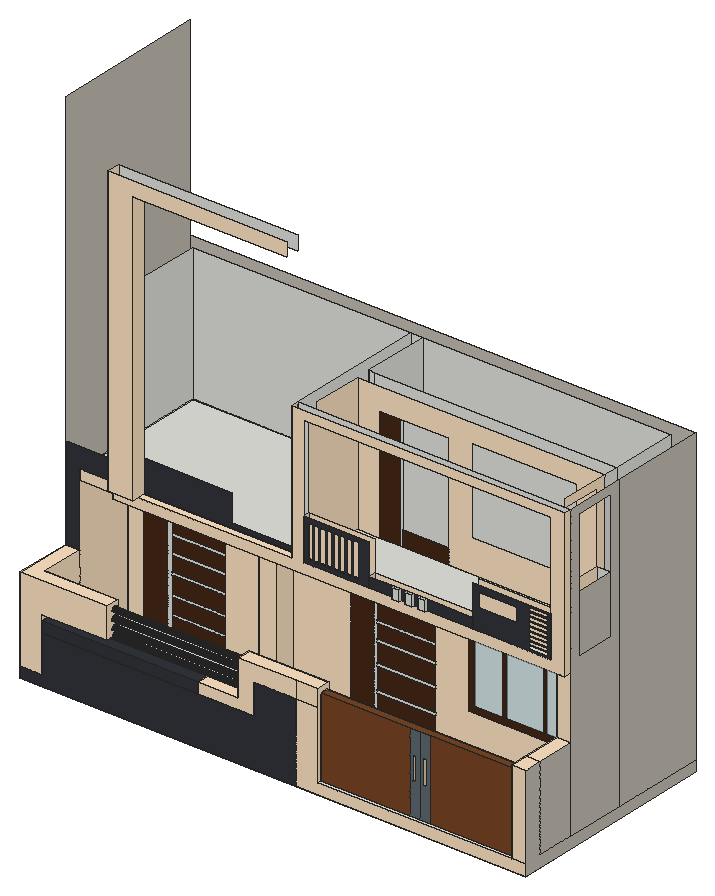
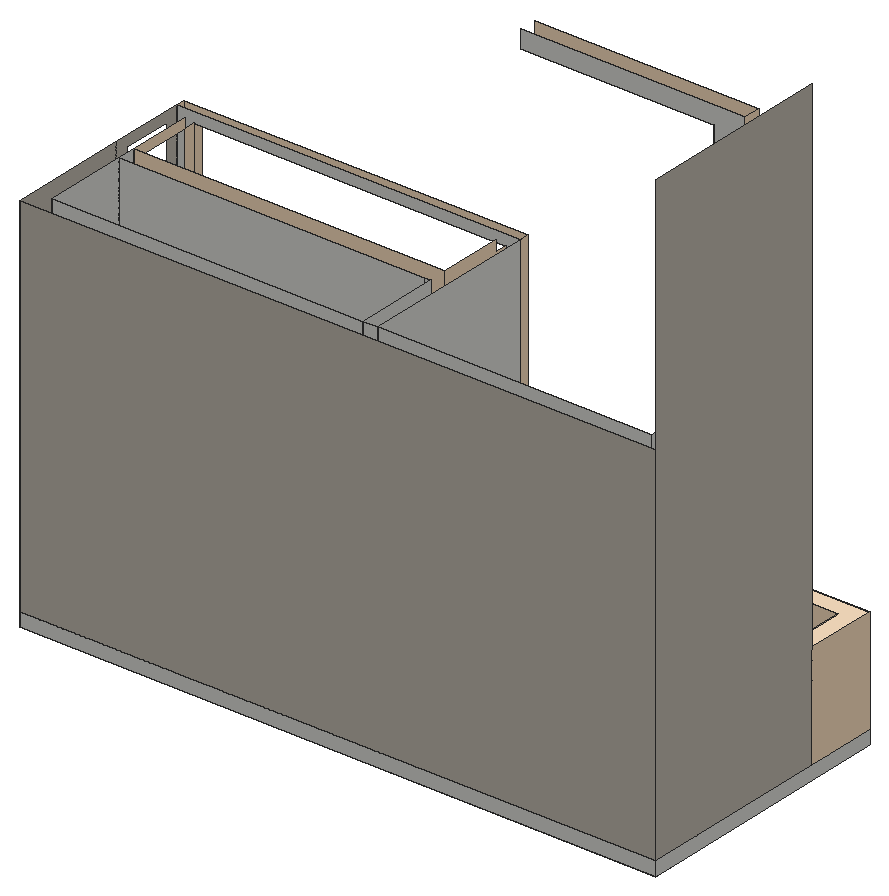
# SketchUp Ruby script. Lengths in inches.
U = 1.inch
M = Sketchup.active_model
def pt(a) = Geom::Point3d.new(a.map { |v| v * U })
def face(e, loops, mat)
  f = e.add_face(loops[0].map { |a| pt(a) })
  loops[1..].each { |l| e.add_face(l.map { |a| pt(a) }).erase! }
  f.material = f.back_material = mat if mat
  f
end
# faces: each face lists its corners as indices into pts; further lists are holes
def faces(e, pts, list, mat = nil) = list.each { |f| face(e, (f[0].is_a?(Array) ? f : [f]).map { |l| l.map { |i| pts[i] } }, mat) }
# xy, xz, yz: faces in a plane at the given z, y or x. An outline is a flat list of corners, or four numbers for a rectangle; further outlines are holes
def ring(l) = l.size == 4 ? [[l[0], l[1]], [l[2], l[1]], [l[2], l[3]], [l[0], l[3]]] : l.each_slice(2).to_a
def flat(e, list, mat, &to3) = list.each { |f| face(e, (f[0].is_a?(Array) ? f : [f]).map { |l| ring(l).map { |u, v| to3.(u, v) } }, mat) }
def xy(e, z, list, mat = nil) = flat(e, list, mat) { |x, y| [x, y, z] }
def xz(e, y, list, mat = nil) = flat(e, list, mat) { |x, z| [x, y, z] }
def yz(e, x, list, mat = nil) = flat(e, list, mat) { |y, z| [x, y, z] }
def lines(e, pts, list) = list.each { |a, b| e.add_line(pt(pts[a]), pt(pts[b])) }
# prism: a flat outline (further loops are holes) pulled along v
def prism(e, loops, v, mat = nil)
  f = face(e, loops, mat); d = Geom::Vector3d.new(v.map { |x| x * U })
  f.pushpull(f.normal.samedirection?(d) ? d.length : -d.length)
end
def box(e, o, s, mat = nil) = prism(e, [[o, [o[0] + s[0], o[1], o[2]], [o[0] + s[0], o[1] + s[1], o[2]], [o[0], o[1] + s[1], o[2]]]], [0, 0, s[2]], mat)
def at(x, y, z, deg = 0) = Geom::Transformation.translation(pt([x, y, z])) * Geom::Transformation.rotation(ORIGIN, Z_AXIS, deg.degrees)
def axes(o, x, y, z) = Geom::Transformation.new([*x, 0, *y, 0, *z, 0, *pt(o).to_a, 1])
def part(name) = M.definitions.add(name)
# library, detail: a bought-in or finely detailed component or shape, given as its bounding box
def library(name, o, s) = part(name).tap { |d| box(d.entities, o, s) }
def detail(e, o, s) = box(e.add_group.entities, o, s)
def put(e, d, t, mat = nil) = e.add_instance(d, t).tap { |i| i.material = mat if mat }
def group(e, t, mat = nil) = e.add_group.tap { |g| g.transformation = t; g.material = mat if mat }.entities
root = M.entities
M.materials.add("[0012_Bisque]").color = [255, 228, 196]
M.materials.add("[Color M08]").color = [30, 30, 30]
M.materials.add("[Field Rectangle Tile]").color = [196, 189, 179]
M.materials.add("[Formica Laminate Dark]").color = [50, 53, 60]
M.materials.add("[Formica Laminate Light]").color = [213, 189, 164]
M.materials.add("[Formica Speckled Grey]").color = [94, 105, 111]
M.materials.add("[Translucent Glass Safety]").color = [204, 235, 244]
M.materials["[Translucent Glass Safety]"].alpha = 0.5
M.materials.add("[Wood Veneer 01]").color = [68, 40, 21]
M.materials.add("[Wood Veneer 01]1").color = [120, 70, 37]
xy(root,0,[[24.6875,0,439.21,174.44]])
xy(root,9,[[24.6875,0,24.6875,46.73,36.15,46.73,36.15,11.46,42.39,11.46,42.39,0],[268.84,0,427.75,3.26],[268.84,3.26,427.75,9.44],[268.84,9.44,427.75,11.46],[36.15,11.46,427.75,11.46,427.75,96.17,171.86,96.17,171.86,78.99,157.61,78.99,157.61,96.17,36.15,96.17],
  [427.75,15.01,439.21,46.73],[24.6875,46.73,24.6875,174.44,439.21,174.44,439.21,96.17,427.75,96.17,427.75,162.99,36.15,162.99,36.15,46.73],[427.75,46.73,439.21,96.17],[157.61,78.99,171.86,96.17],[36.15,96.17,427.75,107.95],
  [36.15,107.95,427.75,162.99]])
xy(root,39.88,[[42.39,0,170.3,11.46],[170.3,0,216.09,11.46]])
xy(root,48.39,[[170.3,0,203.55,11.46]],"[0012_Bisque]")
xy(root,48.39,[[42.39,0,170.3,11.46]],"[Formica Laminate Dark]")
xy(root,52.77,[[42.39,0,95.7,11.46]])
xy(root,73.625,[[268.84,3.26,427.75,9.44]],"[Wood Veneer 01]1")
xy(root,77.8125,[[24.6875,0,95.7,0,95.7,11.46,36.15,11.46,36.15,46.73,24.6875,46.73],[203.55,0,268.84,11.46],[427.75,0,439.21,15.01],[427.75,15.01,439.21,46.73]],"[0012_Bisque]")
xy(root,129,[[36.15,96.17,427.75,107.95],[36.15,107.95,427.75,162.99]])
xy(root,129,[[68.38,40.67,68.38,46.73,36.15,46.73,36.15,96.17,157.61,96.17,157.61,78.99,171.86,78.99,171.86,96.17,427.75,96.17,427.75,40.67],[427.75,40.67,439.21,46.73]],"[0012_Bisque]")
xy(root,137.375,[[68.38,35.36,89.06,40.67],[298.64,38.8,304.69,40.67],[309.14,38.8,315.19,40.67],[319.64,38.8,325.69,40.67],[68.38,40.67,89.06,46.73],
  [224.52,40.67,278.51,46.73],[278.51,40.67,363.63,46.73],[363.63,40.67,427.75,46.73],[36.15,46.73,215,162.99],[224.52,46.73,427.75,96.17],
  [427.75,54.79,439.21,87.8],[228.84,96.17,427.75,107.95],[224.52,107.95,427.75,162.99]])
xy(root,137.375,[[89.06,40.67,215,46.73]],"[0012_Bisque]")
xz(root,0,[[250.74,0,439.21,0,439.21,9,268.84,9,268.84,64.2,250.74,64.2],[24.6875,9,42.39,9,42.39,52.77,95.7,52.77,95.7,77.8125,24.6875,77.8125],[427.75,9,439.21,77.8125],[170.3,39.88,216.09,39.88,216.09,64.2,250.74,64.2,250.74,77.8125,203.55,77.8125,203.55,48.39,170.3,48.39],[250.74,64.2,268.84,77.8125]],"[0012_Bisque]")
xz(root,0,[[24.6875,0,250.74,0,250.74,64.2,216.09,64.2,216.09,39.88,42.39,39.88,42.39,9,24.6875,9],[42.39,39.88,170.3,48.39]],"[Formica Laminate Dark]")
xz(root,3.26,[[344.53,35.39,346.35,54.45],[353.35,35.39,355.16,54.45]],"[Formica Laminate Light]")
xz(root,3.26,[[[341.6875,9,350.3,73.625],[344.53,35.39,346.35,54.45]],[[350.3,9,358.91,73.625],[353.35,35.39,355.16,54.45]]],"[Formica Speckled Grey]")
xz(root,3.26,[[268.84,9,341.6875,73.625],[358.91,9,427.75,73.625]],"[Wood Veneer 01]1")
xz(root,9.44,[[268.84,9,427.75,73.625]],"[Wood Veneer 01]1")
xz(root,11.46,[[36.15,9,36.15,77.8125,95.7,77.8125,95.7,52.77,42.39,52.77,42.39,9],[42.39,9,250.74,39.88],[250.74,9,250.74,64.2,216.09,64.2,216.09,39.88,170.3,39.88,170.3,48.39,203.55,48.39,203.55,77.8125,268.84,77.8125,268.84,9],[42.39,39.88,170.3,48.39],[216.09,39.88,250.74,64.2]],"[0012_Bisque]")
xz(root,35.36,[[68.38,137.375,89.06,137.375,89.06,360.6,215,360.6,215,372.25,68.38,372.25]],"[0012_Bisque]")
xz(root,38.8,[[298.64,137.375,304.69,145.875],[309.14,137.375,315.19,145.875],[319.64,137.375,325.69,145.875]])
xz(root,40.67,[[298.64,137.375,304.69,145.875],[309.14,137.375,315.19,145.875],[319.64,137.375,325.69,145.875]])
xz(root,40.67,[[[68.38,129,439.21,129,439.21,249,215,249,215,137.375,68.38,137.375],[224.52,137.375,427.75,242.43]]],"[0012_Bisque]")
xz(root,40.67,[[[224.52,137.375,278.51,171.25],[227.93,140.39,232.05,168.02],[233.37,140.39,237.49,168.02],[238.43,140.39,242.55,168.02],[244.05,140.39,248.18,168.02],[249.43,140.39,253.55,168.02],[254.74,140.39,258.87,168.02],[260.12,140.39,264.24,168.02],[265.49,140.39,269.62,168.02]],[278.51,137.375,298.64,145.875],[304.69,137.375,309.14,145.875],[315.19,137.375,319.64,145.875],[325.69,137.375,363.63,145.875],
  [[363.63,137.375,427.75,171.25],[368.61,154.46,399.74,166.58],[409.26,166.78,424.76,169.97],[409.2,163.09,424.7,166.28],[409.2,159.47,424.7,162.65],[409.2,155.84,424.7,159.03],[409.2,152.34,424.7,155.53],[409.2,148.53,424.7,151.72],[409.2,145.15,424.7,148.34],[409.2,141.72,424.7,144.9],[409.2,138.47,424.7,141.65]]],"[Formica Laminate Dark]")
xz(root,46.73,[[24.6875,9,36.15,77.8125],[[68.38,129,68.38,137.375,215,137.375,215,249,439.21,249,439.21,129,215,129,215,136.36,161.14,136.36,161.14,129],[224.52,137.375,427.75,242.43]],[68.38,137.375,89.06,137.375,89.06,360.6,215,360.6,215,372.25,68.38,372.25]])
xz(root,46.73,[[427.75,77.8125,439.21,129],[36.15,129,68.38,137.375],[224.52,137.375,278.51,171.25],[278.51,137.375,363.63,145.875],[363.63,137.375,427.75,171.25]],"[0012_Bisque]")
xz(root,46.73,[[24.6875,77.8125,36.15,77.8125,36.15,137.375,68.38,137.375,68.38,153.73,24.6875,153.73],[89.06,137.375,215,137.375,215,141.51,161.14,141.51,161.14,163.67,89.06,163.67]],"[Formica Laminate Dark]")
xz(root,54.79,[[427.75,137.375,439.21,185.0625]])
xz(root,78.99,[[157.61,9,171.86,129]],"[0012_Bisque]")
xz(root,87.8,[[427.75,137.375,439.21,185.0625]])
xz(root,96.17,[[68.76,9,71.96,111.5625],[157.61,9,171.86,129],[238.3,9,240.55,113.3125],[71.96,19.84,116.54,22.0625],[240.55,22.59,288.875,24.76],
  [71.96,34.28,116.54,36.5],[240.55,42.42,288.875,44.59],[71.96,50.59,116.54,52.8125],[240.55,60.09,288.875,62.26],[71.96,64.9,116.54,67.125],
  [240.55,74.46,288.875,76.63],[71.96,79.09,116.54,81.3125],[240.55,94.27,288.875,96.44],[71.96,94.65,116.54,96.875],[259.77,137.375,262.03,230.51]])
xz(root,96.17,[[36.15,9,48.29,9,48.29,111.5625,116.54,111.5625,116.54,9,157.61,9,157.61,129,36.15,129],[[171.86,9,219.3125,9,219.3125,113.3125,288.875,113.3125,288.875,9,427.75,9,427.75,129,171.86,129],[315.74,35.89,409.24,113.76]],[[224.52,137.375,241.9,137.375,241.9,230.51,299.47,230.51,299.47,137.375,427.75,137.375,427.75,249,224.52,249],[318.53,163.84,404.47,234.09]]],"[0012_Bisque]")
xz(root,96.17,[[320.85,41,343.74,108.65],[346.68,41,377.11,108.65],[380.05,41,404.13,108.65]],"[Translucent Glass Safety]")
xz(root,96.17,[[48.29,9,68.76,111.5625],[71.96,9,116.54,19.84],[219.3125,9,238.3,113.3125],[240.55,9,288.875,22.59],[71.96,22.0625,116.54,34.28],
  [240.55,24.76,288.875,42.42],[[315.74,35.89,409.24,113.76],[320.85,41,404.13,108.65]],[71.96,36.5,116.54,50.59],[343.74,41,346.68,108.65],[377.11,41,380.05,108.65],
  [240.55,44.59,288.875,60.09],[71.96,52.8125,116.54,64.9],[240.55,62.26,288.875,74.46],[71.96,67.125,116.54,79.09],[240.55,76.63,288.875,94.27],
  [71.96,81.3125,116.54,94.65],[240.55,96.44,288.875,113.3125],[71.96,96.875,116.54,111.5625],[241.9,137.375,259.77,230.51],[262.03,137.375,299.47,150.42]],"[Wood Veneer 01]")
xz(root,107.95,[[36.15,9,427.75,129],[224.52,137.375,228.84,249],[228.84,137.375,427.75,249]])
xz(root,162.99,[[36.15,9,427.75,129],[36.15,129,427.75,129,427.75,137.375,224.52,137.375,224.52,249,215,249,215,137.375,36.15,137.375],[36.15,137.375,215,249],[224.52,137.375,427.75,249]])
xz(root,174.44,[[24.6875,0,439.21,9]])
xz(root,174.44,[[24.6875,9,439.21,249]],"[Field Rectangle Tile]")
yz(root,24.6875,[[0,0,174.44,9]])
yz(root,24.6875,[[0,9,46.73,77.8125]],"[0012_Bisque]")
yz(root,24.6875,[[46.73,9,174.44,406.75]],"[Field Rectangle Tile]")
yz(root,36.15,[[96.17,9,107.95,129],[107.95,9,162.99,129],[46.73,129,107.95,137.375],[107.95,129,162.99,137.375],[107.95,137.375,162.99,249]])
yz(root,36.15,[[11.46,9,46.73,77.8125],[46.73,9,96.17,129]],"[0012_Bisque]")
yz(root,42.39,[[0,9,11.46,39.88],[0,39.88,11.46,48.39]])
yz(root,42.39,[[0,48.39,11.46,52.77]],"[0012_Bisque]")
yz(root,68.38,[[40.67,129,46.73,137.375],[35.36,137.375,46.73,372.25]],"[0012_Bisque]")
yz(root,89.06,[[35.36,137.375,46.73,360.6]],"[0012_Bisque]")
yz(root,95.7,[[6.99,51.16,6.49,51.21,6.01,51.39,5.6,51.6875,5.28,52.08,5.07,52.54,5.04,52.77,8.83,52.77,8.81,52.66,8.64,52.1875,8.34,51.78,7.95,51.45,7.49,51.25],[5.04,52.77,8.83,52.77,8.86,53.16,8.78,53.66,8.57,54.12,8.25,54.51,7.84,54.81,7.37,54.99,6.86,55.04,6.37,54.95,5.91,54.75,5.51,54.42,5.22,54.01,5.04,53.54,4.99,53.04]])
yz(root,95.7,[[[0,52.77,5.04,52.77,4.99,53.04,5.04,53.54,5.22,54.01,5.51,54.42,5.91,54.75,6.37,54.95,6.86,55.04,7.37,54.99,7.84,54.81,8.25,54.51,8.57,54.12,8.78,53.66,8.86,53.16,8.83,52.77,11.46,52.77,11.46,77.8125,0,77.8125],[6.99,71.16,6.49,71.21,6.01,71.39,5.6,71.6875,5.28,72.08,5.07,72.54,4.99,73.04,5.04,73.54,5.22,74.01,5.51,74.42,5.91,74.75,6.37,74.95,6.86,75.04,7.37,74.99,7.84,74.81,8.25,74.51,8.57,74.12,8.78,73.66,8.86,73.16,8.81,72.66,8.64,72.1875,8.34,71.78,7.95,71.45,7.49,71.25],[6.76,64.58,6.26,64.63,5.78,64.81,5.37,65.1,5.05,65.49,4.84,65.95,4.76,66.45,4.8125,66.95,4.99,67.43,5.28,67.84,5.67,68.16,6.14,68.37,6.63,68.45,7.14,68.4,7.61,68.22,8.02,67.93,8.34,67.54,8.55,67.08,8.63,66.58,8.58,66.07,8.41,65.6,8.11,65.19,7.72,64.87,7.26,64.66],[6.99,57.48,6.49,57.53,6.01,57.7,5.6,58,5.28,58.39,5.07,58.85,4.99,59.35,5.04,59.85,5.22,60.33,5.51,60.74,5.91,61.06,6.37,61.27,6.86,61.35,7.37,61.3,7.84,61.12,8.25,60.83,8.57,60.44,8.78,59.97,8.86,59.48,8.81,58.97,8.64,58.5,8.34,58.09,7.95,57.77,7.49,57.56]]],"[0012_Bisque]")
yz(root,157.61,[[78.99,9,96.17,129]],"[0012_Bisque]")
yz(root,170.3,[[0,39.88,11.46,48.39]])
yz(root,171.86,[[78.99,9,96.17,129]],"[0012_Bisque]")
yz(root,203.55,[[6.99,51.16,7.49,51.25,7.95,51.45,8.34,51.78,8.64,52.1875,8.81,52.66,8.86,53.16,8.78,53.66,8.57,54.12,8.25,54.51,7.84,54.81,7.37,54.99,6.86,55.04,6.37,54.95,5.91,54.75,5.51,54.42,5.22,54.01,5.04,53.54,4.99,53.04,5.07,52.54,5.28,52.08,5.6,51.6875,6.01,51.39,6.49,51.21],[6.99,57.48,7.49,57.56,7.95,57.77,8.34,58.09,8.64,58.5,8.81,58.97,8.86,59.48,8.78,59.97,8.57,60.44,8.25,60.83,7.84,61.12,7.37,61.3,6.86,61.35,6.37,61.27,5.91,61.06,5.51,60.74,5.22,60.33,5.04,59.85,4.99,59.35,5.07,58.85,5.28,58.39,5.6,58,6.01,57.7,6.49,57.53],[6.76,64.58,7.26,64.66,7.72,64.87,8.11,65.19,8.41,65.6,8.58,66.07,8.63,66.58,8.55,67.08,8.34,67.54,8.02,67.93,7.61,68.22,7.14,68.4,6.63,68.45,6.14,68.37,5.67,68.16,5.28,67.84,4.99,67.43,4.8125,66.95,4.76,66.45,4.84,65.95,5.05,65.49,5.37,65.1,5.78,64.81,6.26,64.63],[6.99,71.16,7.49,71.25,7.95,71.45,8.34,71.78,8.64,72.1875,8.81,72.66,8.86,73.16,8.78,73.66,8.57,74.12,8.25,74.51,7.84,74.81,7.37,74.99,6.86,75.04,6.37,74.95,5.91,74.75,5.51,74.42,5.22,74.01,5.04,73.54,4.99,73.04,5.07,72.54,5.28,72.08,5.6,71.6875,6.01,71.39,6.49,71.21]])
yz(root,203.55,[[[0,48.39,11.46,77.8125],[6.99,51.16,7.49,51.25,7.95,51.45,8.34,51.78,8.64,52.1875,8.81,52.66,8.86,53.16,8.78,53.66,8.57,54.12,8.25,54.51,7.84,54.81,7.37,54.99,6.86,55.04,6.37,54.95,5.91,54.75,5.51,54.42,5.22,54.01,5.04,53.54,4.99,53.04,5.07,52.54,5.28,52.08,5.6,51.6875,6.01,51.39,6.49,51.21],[6.76,64.58,7.26,64.66,7.72,64.87,8.11,65.19,8.41,65.6,8.58,66.07,8.63,66.58,8.55,67.08,8.34,67.54,8.02,67.93,7.61,68.22,7.14,68.4,6.63,68.45,6.14,68.37,5.67,68.16,5.28,67.84,4.99,67.43,4.8125,66.95,4.76,66.45,4.84,65.95,5.05,65.49,5.37,65.1,5.78,64.81,6.26,64.63],[6.99,57.48,7.49,57.56,7.95,57.77,8.34,58.09,8.64,58.5,8.81,58.97,8.86,59.48,8.78,59.97,8.57,60.44,8.25,60.83,7.84,61.12,7.37,61.3,6.86,61.35,6.37,61.27,5.91,61.06,5.51,60.74,5.22,60.33,5.04,59.85,4.99,59.35,5.07,58.85,5.28,58.39,5.6,58,6.01,57.7,6.49,57.53],[6.99,71.16,7.49,71.25,7.95,71.45,8.34,71.78,8.64,72.1875,8.81,72.66,8.86,73.16,8.78,73.66,8.57,74.12,8.25,74.51,7.84,74.81,7.37,74.99,6.86,75.04,6.37,74.95,5.91,74.75,5.51,74.42,5.22,74.01,5.04,73.54,4.99,73.04,5.07,72.54,5.28,72.08,5.6,71.6875,6.01,71.39,6.49,71.21]]],"[0012_Bisque]")
yz(root,215,[[46.73,137.375,162.99,249]])
yz(root,215,[[40.67,137.375,46.73,249]],"[0012_Bisque]")
yz(root,216.09,[[0,39.88,11.46,64.2]])
yz(root,224.52,[[40.67,137.375,46.73,171.25],[107.95,137.375,162.99,249]])
yz(root,224.52,[[46.73,137.375,96.17,137.375,96.17,249,54.79,249,54.79,242.43,46.73,242.43]],"[0012_Bisque]")
yz(root,250.74,[[0,39.88,11.46,64.2]])
yz(root,268.84,[[3.26,9,9.44,73.625]])
yz(root,268.84,[[0,9,3.26,9,3.26,73.625,9.44,73.625,9.44,9,11.46,9,11.46,77.8125,0,77.8125]],"[0012_Bisque]")
yz(root,278.51,[[40.67,137.375,46.73,145.875]])
yz(root,298.64,[[38.8,137.375,40.67,145.875]])
yz(root,304.69,[[38.8,137.375,40.67,145.875]])
yz(root,309.14,[[38.8,137.375,40.67,145.875]])
yz(root,315.19,[[38.8,137.375,40.67,145.875]])
yz(root,319.64,[[38.8,137.375,40.67,145.875]])
yz(root,325.69,[[38.8,137.375,40.67,145.875]])
yz(root,363.63,[[40.67,137.375,46.73,145.875]])
yz(root,427.75,[[96.17,9,107.95,129],[107.95,9,162.99,129],[96.17,129,107.95,137.375],[107.95,129,162.99,137.375],[40.67,137.375,46.73,171.25],
  [96.17,137.375,107.95,249],[107.95,137.375,162.99,249]])
yz(root,427.75,[[0,9,0,77.8125,11.46,77.8125,11.46,9,9.44,9,9.44,73.625,3.26,73.625,3.26,9],[11.46,9,11.46,77.8125,46.73,77.8125,46.73,129,96.17,129,96.17,9],[46.73,137.375,54.79,242.43],[54.79,137.375,87.8,185.0625],[87.8,137.375,87.8,242.43,54.79,242.43,54.79,249,96.17,249,96.17,137.375]],"[0012_Bisque]")
yz(root,439.21,[[40.67,129,46.73,249]],"[0012_Bisque]")
yz(root,439.21,[[0,0,174.44,0,174.44,9,15.01,9,15.01,77.8125,0,77.8125],[15.01,9,46.73,77.8125],[[46.73,9,96.17,249],[54.79,137.375,87.8,242.43]],[96.17,9,174.44,249],[54.79,137.375,87.8,185.0625]],"[Field Rectangle Tile]")
p = [[203.55,6.49,51.21],[203.55,6.01,51.39],[95.7,6.01,51.39],[95.7,6.49,51.21],[203.55,6.99,51.16],[95.7,6.99,51.16],
  [203.55,7.49,51.25],[95.7,7.49,51.25],[203.55,7.95,51.45],[95.7,7.95,51.45],[203.55,5.6,51.6875],[95.7,5.6,51.6875],
  [203.55,8.34,51.78],[95.7,8.34,51.78],[203.55,5.28,52.08],[95.7,5.28,52.08],[203.55,8.64,52.1875],[95.7,8.64,52.1875],
  [203.55,5.07,52.54],[95.7,5.07,52.54],[203.55,8.81,52.66],[95.7,8.81,52.66],[203.55,4.99,53.04],[95.7,4.99,53.04],
  [95.7,5.04,52.77],[203.55,8.86,53.16],[95.7,8.83,52.77],[95.7,8.86,53.16],[203.55,5.04,53.54],[95.7,5.04,53.54],
  [203.55,8.78,53.66],[95.7,8.78,53.66],[203.55,5.22,54.01],[95.7,5.22,54.01],[203.55,8.57,54.12],[95.7,8.57,54.12],
  [203.55,5.51,54.42],[95.7,5.51,54.42],[203.55,8.25,54.51],[95.7,8.25,54.51],[203.55,5.91,54.75],[95.7,5.91,54.75],
  [203.55,7.84,54.81],[95.7,7.84,54.81],[203.55,6.37,54.95],[95.7,6.37,54.95],[203.55,7.37,54.99],[95.7,7.37,54.99],
  [203.55,6.86,55.04],[95.7,6.86,55.04],[203.55,6.49,57.53],[203.55,6.01,57.7],[95.7,6.01,57.7],[95.7,6.49,57.53],
  [203.55,6.99,57.48],[95.7,6.99,57.48],[203.55,7.49,57.56],[95.7,7.49,57.56],[203.55,7.95,57.77],[95.7,7.95,57.77],
  [203.55,5.6,58],[95.7,5.6,58],[203.55,8.34,58.09],[95.7,8.34,58.09],[203.55,5.28,58.39],[95.7,5.28,58.39],
  [203.55,8.64,58.5],[95.7,8.64,58.5],[203.55,5.07,58.85],[95.7,5.07,58.85],[203.55,8.81,58.97],[95.7,8.81,58.97],
  [203.55,4.99,59.35],[95.7,4.99,59.35],[203.55,8.86,59.48],[95.7,8.86,59.48],[203.55,5.04,59.85],[95.7,5.04,59.85],
  [203.55,8.78,59.97],[95.7,8.78,59.97],[203.55,5.22,60.33],[95.7,5.22,60.33],[203.55,8.57,60.44],[95.7,8.57,60.44],
  [203.55,5.51,60.74],[95.7,5.51,60.74],[203.55,8.25,60.83],[95.7,8.25,60.83],[203.55,5.91,61.06],[95.7,5.91,61.06],
  [203.55,7.84,61.12],[95.7,7.84,61.12],[203.55,6.37,61.27],[95.7,6.37,61.27],[203.55,7.37,61.3],[95.7,7.37,61.3],
  [203.55,6.86,61.35],[95.7,6.86,61.35],[203.55,6.26,64.63],[203.55,5.78,64.81],[95.7,5.78,64.81],[95.7,6.26,64.63],
  [203.55,6.76,64.58],[95.7,6.76,64.58],[203.55,7.26,64.66],[95.7,7.26,64.66],[203.55,7.72,64.87],[95.7,7.72,64.87],
  [203.55,5.37,65.1],[95.7,5.37,65.1],[203.55,8.11,65.19],[95.7,8.11,65.19],[203.55,5.05,65.49],[95.7,5.05,65.49],
  [203.55,8.41,65.6],[95.7,8.41,65.6],[203.55,4.84,65.95],[95.7,4.84,65.95],[203.55,8.58,66.07],[95.7,8.58,66.07],
  [203.55,4.76,66.45],[95.7,4.76,66.45],[203.55,8.63,66.58],[95.7,8.63,66.58],[203.55,4.8125,66.95],[95.7,4.8125,66.95],
  [203.55,8.55,67.08],[95.7,8.55,67.08],[203.55,4.99,67.43],[95.7,4.99,67.43],[203.55,8.34,67.54],[95.7,8.34,67.54],
  [203.55,5.28,67.84],[95.7,5.28,67.84],[203.55,8.02,67.93],[95.7,8.02,67.93],[203.55,5.67,68.16],[95.7,5.67,68.16],
  [203.55,7.61,68.22],[95.7,7.61,68.22],[203.55,6.14,68.37],[95.7,6.14,68.37],[203.55,7.14,68.4],[95.7,7.14,68.4],
  [203.55,6.63,68.45],[95.7,6.63,68.45],[203.55,6.49,71.21],[203.55,6.01,71.39],[95.7,6.01,71.39],[95.7,6.49,71.21],
  [203.55,6.99,71.16],[95.7,6.99,71.16],[203.55,7.49,71.25],[95.7,7.49,71.25],[203.55,7.95,71.45],[95.7,7.95,71.45],
  [203.55,5.6,71.6875],[95.7,5.6,71.6875],[203.55,8.34,71.78],[95.7,8.34,71.78],[203.55,5.28,72.08],[95.7,5.28,72.08],
  [203.55,8.64,72.1875],[95.7,8.64,72.1875],[203.55,5.07,72.54],[95.7,5.07,72.54],[203.55,8.81,72.66],[95.7,8.81,72.66],
  [203.55,4.99,73.04],[95.7,4.99,73.04],[203.55,8.86,73.16],[95.7,8.86,73.16],[203.55,5.04,73.54],[95.7,5.04,73.54],
  [203.55,8.78,73.66],[95.7,8.78,73.66],[203.55,5.22,74.01],[95.7,5.22,74.01],[203.55,8.57,74.12],[95.7,8.57,74.12],
  [203.55,5.51,74.42],[95.7,5.51,74.42],[203.55,8.25,74.51],[95.7,8.25,74.51],[203.55,5.91,74.75],[95.7,5.91,74.75],
  [203.55,7.84,74.81],[95.7,7.84,74.81],[203.55,6.37,74.95],[95.7,6.37,74.95],[203.55,7.37,74.99],[95.7,7.37,74.99],
  [203.55,6.86,75.04],[95.7,6.86,75.04]]
faces(root,p,[[0,1,2,3],[4,0,3,5],[6,4,5,7],[8,6,7,9],[1,10,11,2],[12,8,9,13],[10,14,15,11],[16,12,13,17],
  [14,18,19,15],[20,16,17,21],[18,22,23,24,19],[25,20,21,26,27],[22,28,29,23],[30,25,27,31],[28,32,33,29],[34,30,31,35],
  [32,36,37,33],[38,34,35,39],[36,40,41,37],[42,38,39,43],[40,44,45,41],[46,42,43,47],[44,48,49,45],[48,46,47,49],
  [50,51,52,53],[54,50,53,55],[56,54,55,57],[58,56,57,59],[51,60,61,52],[62,58,59,63],[60,64,65,61],[66,62,63,67],
  [64,68,69,65],[70,66,67,71],[68,72,73,69],[74,70,71,75],[72,76,77,73],[78,74,75,79],[76,80,81,77],[82,78,79,83],
  [80,84,85,81],[86,82,83,87],[84,88,89,85],[90,86,87,91],[88,92,93,89],[94,90,91,95],[92,96,97,93],[96,94,95,97],
  [98,99,100,101],[102,98,101,103],[104,102,103,105],[106,104,105,107],[99,108,109,100],[110,106,107,111],[108,112,113,109],[114,110,111,115],
  [112,116,117,113],[118,114,115,119],[116,120,121,117],[122,118,119,123],[120,124,125,121],[126,122,123,127],[124,128,129,125],[130,126,127,131],
  [128,132,133,129],[134,130,131,135],[132,136,137,133],[138,134,135,139],[136,140,141,137],[142,138,139,143],[140,144,145,141],[144,142,143,145],
  [146,147,148,149],[150,146,149,151],[152,150,151,153],[154,152,153,155],[147,156,157,148],[158,154,155,159],[156,160,161,157],[162,158,159,163],
  [160,164,165,161],[166,162,163,167],[164,168,169,165],[170,166,167,171],[168,172,173,169],[174,170,171,175],[172,176,177,173],[178,174,175,179],
  [176,180,181,177],[182,178,179,183],[180,184,185,181],[186,182,183,187],[184,188,189,185],[190,186,187,191],[188,192,193,189],[192,190,191,193]],"[Color M08]")
